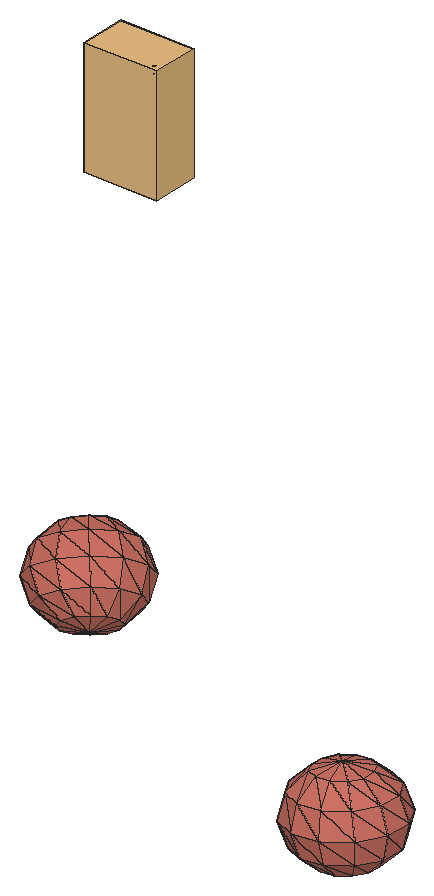
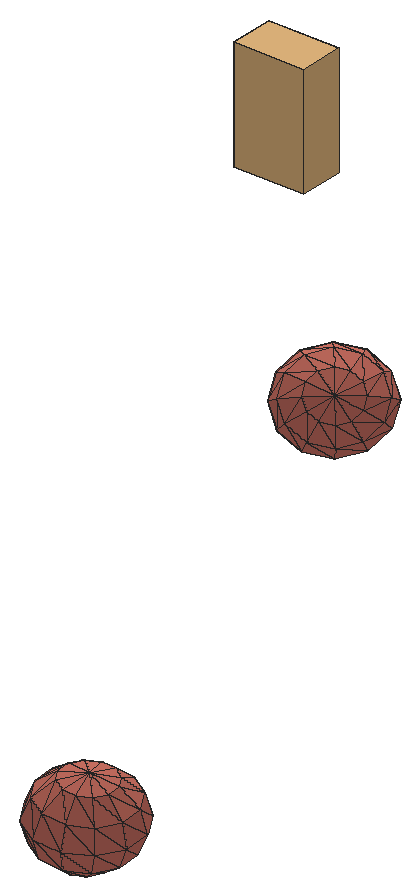
# SketchUp Ruby script. Lengths in inches.
U = 1.inch
M = Sketchup.active_model
def pt(a) = Geom::Point3d.new(a.map { |v| v * U })
def face(e, loops, mat)
  f = e.add_face(loops[0].map { |a| pt(a) })
  loops[1..].each { |l| e.add_face(l.map { |a| pt(a) }).erase! }
  f.material = f.back_material = mat if mat
  f
end
# faces: each face lists its corners as indices into pts; further lists are holes
def faces(e, pts, list, mat = nil) = list.each { |f| face(e, (f[0].is_a?(Array) ? f : [f]).map { |l| l.map { |i| pts[i] } }, mat) }
# xy, xz, yz: faces in a plane at the given z, y or x. An outline is a flat list of corners, or four numbers for a rectangle; further outlines are holes
def ring(l) = l.size == 4 ? [[l[0], l[1]], [l[2], l[1]], [l[2], l[3]], [l[0], l[3]]] : l.each_slice(2).to_a
def flat(e, list, mat, &to3) = list.each { |f| face(e, (f[0].is_a?(Array) ? f : [f]).map { |l| ring(l).map { |u, v| to3.(u, v) } }, mat) }
def xy(e, z, list, mat = nil) = flat(e, list, mat) { |x, y| [x, y, z] }
def xz(e, y, list, mat = nil) = flat(e, list, mat) { |x, z| [x, y, z] }
def yz(e, x, list, mat = nil) = flat(e, list, mat) { |y, z| [x, y, z] }
def lines(e, pts, list) = list.each { |a, b| e.add_line(pt(pts[a]), pt(pts[b])) }
# prism: a flat outline (further loops are holes) pulled along v
def prism(e, loops, v, mat = nil)
  f = face(e, loops, mat); d = Geom::Vector3d.new(v.map { |x| x * U })
  f.pushpull(f.normal.samedirection?(d) ? d.length : -d.length)
end
def box(e, o, s, mat = nil) = prism(e, [[o, [o[0] + s[0], o[1], o[2]], [o[0] + s[0], o[1] + s[1], o[2]], [o[0], o[1] + s[1], o[2]]]], [0, 0, s[2]], mat)
def at(x, y, z, deg = 0) = Geom::Transformation.translation(pt([x, y, z])) * Geom::Transformation.rotation(ORIGIN, Z_AXIS, deg.degrees)
def axes(o, x, y, z) = Geom::Transformation.new([*x, 0, *y, 0, *z, 0, *pt(o).to_a, 1])
def part(name) = M.definitions.add(name)
# library, detail: a bought-in or finely detailed component or shape, given as its bounding box
def library(name, o, s) = part(name).tap { |d| box(d.entities, o, s) }
def detail(e, o, s) = box(e.add_group.entities, o, s)
def put(e, d, t, mat = nil) = e.add_instance(d, t).tap { |i| i.material = mat if mat }
def group(e, t, mat = nil) = e.add_group.tap { |g| g.transformation = t; g.material = mat if mat }.entities
root = M.entities
M.materials.add("green").color = [174, 139, 102]
M.materials.add("vio").color = [206, 114, 100]
c1 = library("3DGeom~53_Defintion",[-197.77,-500,-314.82],[395.54,1000,629.64])
c2 = part("3DGeom~54_Defintion")
p = [[-142.75,-484.5,-308.47],[-174.69,-472.9,-312.45],[-157.62,-477.6,-314.82],[-174.69,-472.9,-312.45],[-142.75,-484.5,-308.47],[-197.77,-474.24,-286.23],
  [-174.69,-472.9,-312.45],[-197.77,-474.24,-286.23],[-189.38,-471.68,-301.98],[-188.9,-487.18,-256.03],[-142.75,-484.5,-308.47],[-156.97,-498.77,-252.06],
  [-156.97,-498.77,-252.06],[-142.75,-484.5,-308.47],[-133.89,-497.43,-278.27],[-142.75,-484.5,-308.47],[-134.07,-491.76,-295.09],[-133.89,-497.43,-278.27],
  [-197.77,-474.24,-286.23],[-142.75,-484.5,-308.47],[-188.9,-487.18,-256.03],[-197.77,-474.24,-286.23],[-188.9,-487.18,-256.03],[-197.59,-479.92,-269.41],
  [-156.97,-498.77,-252.06],[-133.89,-497.43,-278.27],[-142.27,-500,-262.52],[-188.9,-487.18,-256.03],[-156.97,-498.77,-252.06],[-174.04,-494.08,-249.68],
  [187.69,494.74,272.45],[154.39,500,263.8],[138.33,494.89,269.58],[187.69,494.74,272.45],[172.46,499.94,264.85],[154.39,500,263.8],
  [187.69,494.74,272.45],[138.33,494.89,269.58],[128.58,485.99,280.65],[187.69,494.74,272.45],[136.08,466.72,306.16],[151.32,461.51,313.77],
  [187.69,494.74,272.45],[169.38,461.46,314.82],[187.69,494.74,272.45],[185.44,466.57,309.04],[187.69,494.74,272.45],[185.44,466.57,309.04],
  [195.19,475.47,297.97],[187.69,494.74,272.45],[127.76,475.68,294.04],[187.69,494.74,272.45],[195.19,475.47,297.97],[196.01,485.78,284.58],
  [187.69,494.74,272.45],[128.58,485.99,280.65],[127.76,475.68,294.04]]
faces(c2.entities,p,[[0,1,2],[3,4,5],[6,7,8],[9,10,11],[12,13,14],[15,16,17],[18,19,20],[21,22,23],
  [24,25,26],[27,28,29],[30,31,32],[33,34,35],[36,37,38],[39,40,41],[42,41,43],[44,43,45],
  [46,47,48],[49,50,40],[51,52,53],[54,55,56]],"green")
c3 = part("3DGeom~200_Defintion")
p = [[-43.89,-289.91,-363.15],[-189.17,-120.3,-441.1],[-12.44,-14.18,-500],[160.18,-167.375,-431.16],[127.12,130.77,-458.85],[-181.73,142.8125,-434.86],
  [-101.15,226.5,-411.11],[321.33,0,-383.65],[321.33,0,-383.65],[192.11,275.72,-328.68],[-63.63,310.1875,-335.95],[-63.63,310.1875,-335.95],
  [192.11,275.72,-328.68],[-236.2,-334.76,-197.83],[-355.71,-159.14,-297.93],[-236.2,-334.76,-197.83],[-355.71,-159.14,-297.93],[-283.76,81.55,-400.86],
  [-302.32,261.54,-253.21],[-302.32,261.54,-253.21],[113.15,-381.84,-187.89],[113.15,-381.84,-187.89],[289.875,-275.72,-246.79],[289.875,-275.72,-246.79],
  [321.33,0,-383.65],[-63.63,310.1875,-335.95],[-302.32,261.54,-253.21],[-355.71,-159.14,-297.93],[-379.91,59.12,-318.2],[-283.76,81.55,-400.86],
  [-379.91,59.12,-318.2],[-302.32,261.54,-253.21],[289.875,-275.72,-246.79],[321.33,0,-383.65],[429.43,-130.77,-205.64],[429.43,-130.77,-205.64],
  [321.33,0,-383.65],[396.375,167.38,-233.33],[321.33,0,-383.65],[192.11,275.72,-328.68],[396.375,167.38,-233.33],[-53.39,-420.67,-44.72],
  [-236.2,-334.76,-197.83],[-43.89,-289.91,-363.15],[-43.89,-289.91,-363.15],[113.15,-381.84,-187.89],[-79.21,371.45,-229.53],[-63.63,310.1875,-335.95],
  [-302.32,261.54,-253.21],[192.11,275.72,-328.68],[192.11,275.72,-328.68],[165.125,381.84,-144.36],[192.11,275.72,-328.68],[165.125,381.84,-144.36],
  [-467.44,-120.3,-108.85],[-355.71,-159.14,-297.93],[-444.42,81.55,-209.03],[-365.21,-289.91,20.5],[-236.2,-334.76,-197.83],[-365.21,-289.91,20.5],
  [-460,142.8125,-102.62],[-422.48,226.5,-27.46],[-341.9,310.1875,-3.7],[-341.9,310.1875,-3.7],[-239.87,371.45,-37.71],[-302.32,261.54,-253.21],
  [-143.72,393.875,-120.37],[-302.32,261.54,-253.21],[-302.32,261.54,-253.21],[239.87,-371.45,37.71],[289.875,-275.72,-246.79],[289.875,-275.72,-246.79],
  [341.9,-310.19,3.7],[341.9,-310.19,3.7],[289.875,-275.72,-246.79],[494.43,14.18,-75.47],[365.21,289.91,-20.5],[165.125,381.84,-144.36],
  [-494.43,-14.18,75.47],[422.48,-226.5,27.46],[-165.125,-381.83,144.36],[-365.21,-289.91,20.5],[143.72,-393.875,120.37],[365.21,289.91,-20.5],
  [53.39,420.68,44.72],[-396.375,-167.375,233.33],[-365.21,-289.91,20.5],[-429.43,130.77,205.64],[460,-142.8125,102.62],[467.44,120.3,108.85],
  [79.21,-371.45,229.53],[-113.15,381.83,187.89],[-341.9,310.1875,-3.7],[-113.15,381.83,187.89],[-289.875,275.72,246.79],[-289.875,275.72,246.79],
  [236.2,334.75,197.83],[365.21,289.91,-20.5],[236.2,334.75,197.83],[-113.15,381.83,187.89],[-341.9,310.1875,-3.7],[-289.875,275.72,246.79],
  [341.9,-310.19,3.7],[302.32,-261.54,253.21],[302.32,-261.54,253.21],[-192.11,-275.72,328.68],[-365.21,-289.91,20.5],[-165.125,-381.83,144.36],
  [-192.11,-275.72,328.68],[-365.21,-289.91,20.5],[302.32,-261.54,253.21],[236.2,334.75,197.83],[-113.15,381.83,187.89],[-321.32,0,383.65],
  [-321.32,0,383.65],[444.42,-81.55,209.03],[302.32,-261.54,253.21],[355.71,159.14,297.93],[236.2,334.75,197.83],[355.71,159.14,297.93],
  [63.63,-310.1875,335.95],[-192.11,-275.72,328.68],[43.89,289.91,363.15],[-113.15,381.83,187.89],[-289.875,275.72,246.79],[236.2,334.75,197.83],
  [-113.15,381.83,187.89],[43.89,289.91,363.15],[355.71,159.14,297.93],[236.2,334.75,197.83],[-160.18,167.375,431.16],[-429.43,130.77,205.64],
  [-321.32,0,383.65],[-429.43,130.77,205.64],[379.91,-59.12,318.2],[302.32,-261.54,253.21],[355.71,159.14,297.93],[-127.12,-130.77,458.85],
  [-396.375,-167.375,233.33],[-192.11,-275.72,328.68],[-396.375,-167.375,233.33],[101.15,-226.5,411.11],[63.63,-310.1875,335.95],[302.32,-261.54,253.21],
  [181.73,-142.8125,434.86],[302.32,-261.54,253.21],[283.76,-81.55,400.86],[302.32,-261.54,253.21],[283.76,-81.55,400.86],[302.32,-261.54,253.21],
  [379.91,-59.12,318.2],[189.17,120.3,441.1],[379.91,-59.12,318.2],[-192.11,-275.72,328.68],[63.63,-310.1875,335.95],[-192.11,-275.72,328.68],
  [12.44,14.18,500]]
faces(c3.entities,p,[[0,1,2],[0,2,3],[3,2,4],[1,5,2],[2,5,6],[2,6,4],[3,4,7],[8,4,9],
  [4,6,10],[4,11,12],[13,14,1],[15,1,0],[16,17,1],[1,17,5],[5,17,18],[6,5,19],
  [20,0,3],[21,3,22],[23,3,24],[25,6,26],[27,28,17],[29,30,31],[32,33,34],[35,36,37],
  [38,39,40],[41,42,43],[41,44,45],[46,47,48],[49,47,46],[37,50,51],[52,46,53],[54,30,55],
  [54,56,30],[30,56,31],[57,55,58],[59,54,55],[56,60,31],[60,61,31],[61,62,31],[63,64,65],
  [64,66,67],[66,46,68],[69,45,70],[69,71,72],[73,74,35],[35,37,75],[75,37,76],[37,77,76],
  [53,46,66],[78,56,54],[78,60,56],[73,35,79],[79,35,75],[80,42,41],[80,81,42],[82,41,45],
  [82,45,69],[83,53,84],[53,66,84],[84,66,64],[85,54,86],[85,78,54],[87,60,78],[87,61,60],
  [79,75,88],[88,75,89],[75,76,89],[90,80,41],[90,41,82],[91,64,92],[84,64,93],[94,61,87],
  [95,62,61],[89,76,96],[97,84,98],[99,100,101],[69,102,103],[73,79,104],[105,106,107],[108,85,109],
  [79,88,110],[82,69,103],[111,84,112],[113,78,85],[114,87,78],[88,115,116],[88,89,115],[115,89,117],
  [89,118,119],[90,82,103],[120,121,80],[120,80,90],[122,123,124],[125,126,127],[128,129,122],[130,131,132],
  [130,124,133],[115,134,135],[115,136,134],[120,90,103],[137,138,139],[137,132,140],[122,124,130],[141,142,143],
  [144,141,145],[146,144,147],[134,148,149],[150,128,151],[128,122,151],[152,151,146],[141,153,154],[141,137,155],
  [151,122,130],[156,132,137],[156,130,132],[146,156,144],[146,151,156],[144,137,141],[151,130,156],[144,156,137]],"vio")
c4 = part("3DGeom~207_Defintion")
p = [[-123.67,-51.48,-497.34],[-293.26,-262.53,-290.98],[-357.11,-52.125,-367.46],[-91.11,-261.97,-403.46],[-293.26,-262.53,-290.98],[142.89,-37.04,-493.96],
  [-123.1,172.81,-457.96],[-357.11,-52.125,-367.46],[107.75,185.3125,-455.03],[139.75,-249.46,-400.53],[371.18,-12.67,-358.22],[305.45,206.42,-337.48],
  [305.45,206.42,-337.48],[371.18,-12.67,-358.22],[-357.11,-52.125,-367.46],[-325.26,172.25,-345.47],[-89.55,350.79,-295.86],[-325.26,172.25,-345.47],
  [43.74,358.01,-294.17],[43.74,358.01,-294.17],[-89.55,350.79,-295.86],[157.88,370.19,-226.31],[43.74,358.01,-294.17],[157.88,370.19,-226.31],
  [305.45,206.42,-337.48],[-91.11,-261.97,-403.46],[-150.84,-402.59,-136.53],[-293.26,-262.53,-290.98],[-91.11,-261.97,-403.46],[-34.13,-402.27,-201.48],
  [139.75,-249.46,-400.53],[-91.11,-261.97,-403.46],[139.75,-249.46,-400.53],[99.16,-395.05,-199.79],[337.45,-228.36,-282.98],[139.75,-249.46,-400.53],
  [371.18,-12.67,-358.22],[337.45,-228.36,-282.98],[-357.11,-52.125,-367.46],[-293.26,-262.53,-290.98],[-412.55,-251,-93.23],[-494.85,-38.81,-139.11],
  [-325.26,172.25,-345.47],[500,15.09,-126.5],[337.45,-228.36,-282.98],[371.18,-12.67,-358.22],[417.02,230.46,-136.8],[305.45,206.42,-337.48],
  [417.02,230.46,-136.8],[-444.55,183.78,-147.72],[-206.26,350.47,-230.92],[-89.55,350.79,-295.86],[-325.26,172.25,-345.47],[-206.26,350.47,-230.92],
  [222.29,384.07,-110.45],[305.45,206.42,-337.48],[157.88,370.19,-226.31],[417.02,230.46,-136.8],[-89.55,350.79,-295.86],[-206.26,350.47,-230.92],
  [-32,434.78,-54.5],[43.74,358.01,-294.17],[-293.26,-262.53,-290.98],[-219.72,-395.93,-22.36],[-293.26,-262.53,-290.98],[-219.72,-395.93,-22.36],
  [-412.55,-251,-93.23],[337.45,-228.36,-282.98],[213.3,-382.87,-131.92],[449.01,-204.32,-82.31],[213.3,-382.87,-131.92],[-206.26,350.47,-230.92],
  [-275.13,357.125,-116.75],[-275.13,357.125,-116.75],[32,-434.78,54.5],[213.3,-382.87,-131.92],[-500,-15.09,126.5],[-449.01,204.32,82.31],
  [-275.13,357.125,-116.75],[-417.02,-230.46,136.8],[412.55,251,93.23],[417.02,230.46,-136.8],[219.72,395.93,22.36],[417.02,230.46,-136.8],
  [219.72,395.93,22.36],[417.02,230.46,-136.8],[222.29,384.07,-110.45],[-219.72,-395.93,-22.36],[213.3,-382.87,-131.92],[277.71,-368.99,-16.06],
  [277.71,-368.99,-16.06],[494.85,38.81,139.12],[-275.13,357.125,-116.75],[-277.71,368.99,16.06],[-277.71,368.99,16.06],[219.72,395.93,22.36],
  [-219.72,-395.93,-22.36],[-222.29,-384.07,110.45],[-222.29,-384.07,110.45],[444.55,-183.78,147.72],[-213.3,382.87,131.92],[-99.16,395.05,199.79],
  [34.13,402.27,201.48],[150.84,402.59,136.53],[-222.29,-384.07,110.45],[-219.72,-395.93,-22.36],[277.71,-368.99,-16.06],[275.13,-357.125,116.75],
  [275.13,-357.125,116.75],[-277.71,368.99,16.06],[-337.45,228.36,282.98],[-277.71,368.99,16.06],[-337.45,228.36,282.98],[-213.3,382.87,131.92],
  [412.55,251,93.23],[-157.88,-370.19,226.31],[-43.74,-358.01,294.17],[-157.88,-370.19,226.31],[89.55,-350.79,295.86],[-43.74,-358.01,294.17],
  [275.13,-357.125,116.75],[206.26,-350.47,230.92],[206.26,-350.47,230.92],[89.55,-350.79,295.86],[-371.18,12.67,358.22],[-371.18,12.67,358.22],
  [-337.45,228.36,282.98],[293.26,262.53,290.98],[293.26,262.53,290.98],[412.55,251,93.23],[-417.02,-230.46,136.8],[-157.88,-370.19,226.31],
  [325.26,-172.25,345.47],[206.26,-350.47,230.92],[-305.45,-206.42,337.48],[-305.45,-206.42,337.48],[-371.18,12.67,358.22],[-337.45,228.36,282.98],
  [-139.75,249.46,400.53],[-417.02,-230.46,136.8],[-157.88,-370.19,226.31],[-305.45,-206.42,337.48],[357.1,52.125,367.46],[293.26,262.53,290.98],
  [91.11,261.97,403.46],[-305.45,-206.42,337.48],[-157.88,-370.19,226.31],[-43.74,-358.01,294.17],[123.1,-172.81,457.96],[89.55,-350.79,295.86],
  [206.26,-350.47,230.92],[206.26,-350.47,230.92],[325.26,-172.25,345.47],[-337.45,228.36,282.98],[-371.18,12.67,358.22],[-142.9,37.04,493.96],
  [-337.45,228.36,282.98],[-139.75,249.46,400.53],[91.11,261.97,403.46],[357.1,52.125,367.46],[293.26,262.53,290.98],[-107.75,-185.3125,455.03],
  [123.67,51.48,497.34],[325.26,-172.25,345.47],[325.26,-172.25,345.47],[357.1,52.125,367.46],[91.11,261.97,403.46],[357.1,52.125,367.46],
  [-139.75,249.46,400.53],[-139.75,249.46,400.53],[91.11,261.97,403.46]]
faces(c4.entities,p,[[0,1,2],[0,3,4],[5,3,0],[6,0,7],[8,5,0],[8,0,6],[5,9,3],[10,9,5],
  [11,5,8],[12,13,5],[6,14,15],[16,6,17],[18,8,6],[19,6,20],[21,8,22],[23,24,8],
  [25,26,27],[28,29,26],[30,29,31],[32,33,29],[34,33,35],[36,37,9],[38,39,40],[38,40,41],
  [42,38,41],[43,44,45],[46,45,47],[48,43,45],[42,41,49],[50,42,49],[51,52,53],[54,55,56],
  [54,57,55],[58,59,60],[61,58,60],[56,61,60],[62,26,63],[64,65,66],[67,68,33],[69,70,44],
  [43,69,44],[71,49,72],[59,73,60],[54,56,60],[26,29,74],[29,33,74],[33,75,74],[49,41,76],
  [49,76,77],[78,49,77],[41,40,79],[41,79,76],[80,43,81],[82,80,83],[84,85,86],[87,26,74],
  [88,89,74],[69,90,70],[91,69,43],[80,91,43],[92,77,93],[73,94,60],[95,54,60],[40,96,97],
  [40,98,79],[99,90,69],[91,99,69],[94,100,60],[100,101,60],[101,102,60],[103,95,60],[102,103,60],
  [104,105,74],[106,107,74],[99,108,90],[109,77,110],[111,112,113],[103,114,95],[115,104,74],[116,117,74],
  [118,119,74],[120,121,74],[122,123,74],[77,76,124],[77,125,126],[127,91,80],[103,128,129],[130,104,131],
  [132,133,108],[132,108,99],[76,79,134],[76,135,136],[100,137,138],[100,138,101],[102,128,103],[139,140,141],
  [142,99,91],[143,142,91],[142,132,99],[101,138,144],[101,144,102],[102,144,128],[145,146,147],[148,149,150],
  [148,151,152],[153,154,155],[156,155,157],[158,159,160],[145,147,161],[161,147,149],[161,149,148],[154,145,161],
  [162,148,163],[162,164,165],[154,161,155],[166,162,167],[168,155,162],[169,162,170],[155,161,148],[155,148,162]],"vio")
g1 = group(root,at(15.3125,38.42,26.21))
put(g1,c1,axes([-0.37,0.71,9.47],[0,0.00042,0],[0,0,-0.00042],[-0.00042,0,0]),"green")
put(g1,c2,axes([-0.37,0.71,9.47],[0,0.00042,0],[0,0,-0.00042],[-0.00042,0,0]),"green")
g2 = group(root,at(15.3125,38.42,26.21))
put(g2,c3,axes([-0.19,0.26,8.22],[0,0.00039,0],[0,0,-0.00039],[-0.00039,0,0]),"vio")
g3 = group(root,at(15.3125,38.42,26.21))
put(g3,c4,axes([0.03,1.15,7.125],[0,0.00038,0],[0,0,-0.00038],[-0.00038,0,0]),"vio")
